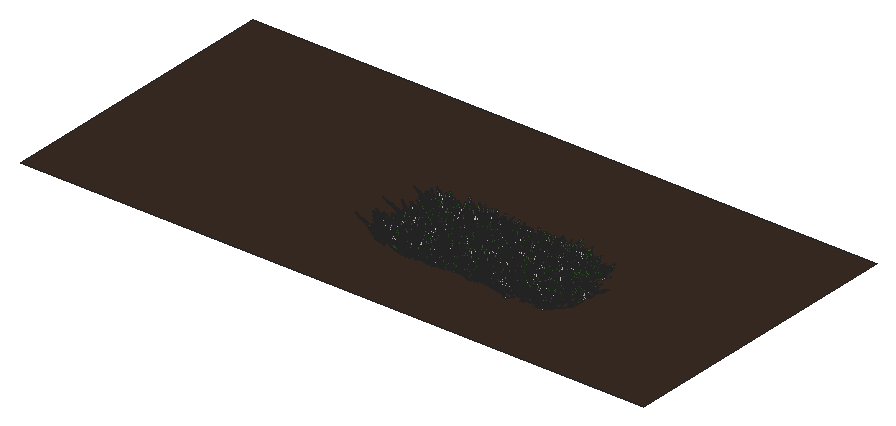
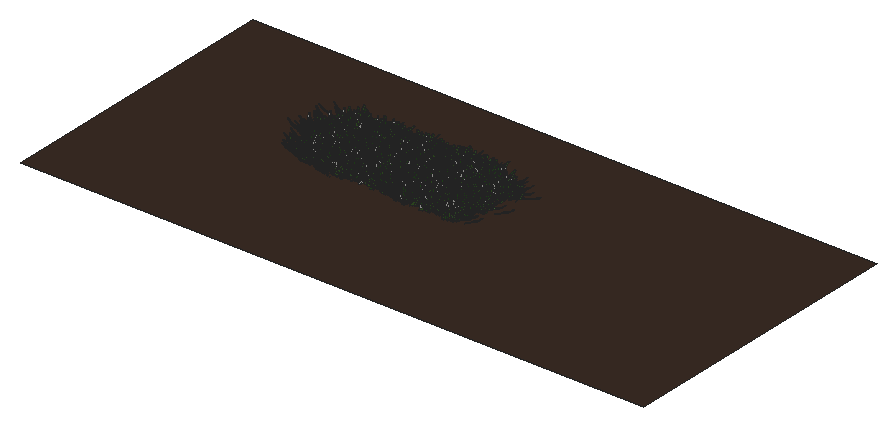
# SketchUp Ruby script. Lengths in inches.
U = 1.inch
M = Sketchup.active_model
def pt(a) = Geom::Point3d.new(a.map { |v| v * U })
def face(e, loops, mat)
  f = e.add_face(loops[0].map { |a| pt(a) })
  loops[1..].each { |l| e.add_face(l.map { |a| pt(a) }).erase! }
  f.material = f.back_material = mat if mat
  f
end
# faces: each face lists its corners as indices into pts; further lists are holes
def faces(e, pts, list, mat = nil) = list.each { |f| face(e, (f[0].is_a?(Array) ? f : [f]).map { |l| l.map { |i| pts[i] } }, mat) }
# xy, xz, yz: faces in a plane at the given z, y or x. An outline is a flat list of corners, or four numbers for a rectangle; further outlines are holes
def ring(l) = l.size == 4 ? [[l[0], l[1]], [l[2], l[1]], [l[2], l[3]], [l[0], l[3]]] : l.each_slice(2).to_a
def flat(e, list, mat, &to3) = list.each { |f| face(e, (f[0].is_a?(Array) ? f : [f]).map { |l| ring(l).map { |u, v| to3.(u, v) } }, mat) }
def xy(e, z, list, mat = nil) = flat(e, list, mat) { |x, y| [x, y, z] }
def xz(e, y, list, mat = nil) = flat(e, list, mat) { |x, z| [x, y, z] }
def yz(e, x, list, mat = nil) = flat(e, list, mat) { |y, z| [x, y, z] }
def lines(e, pts, list) = list.each { |a, b| e.add_line(pt(pts[a]), pt(pts[b])) }
# prism: a flat outline (further loops are holes) pulled along v
def prism(e, loops, v, mat = nil)
  f = face(e, loops, mat); d = Geom::Vector3d.new(v.map { |x| x * U })
  f.pushpull(f.normal.samedirection?(d) ? d.length : -d.length)
end
def box(e, o, s, mat = nil) = prism(e, [[o, [o[0] + s[0], o[1], o[2]], [o[0] + s[0], o[1] + s[1], o[2]], [o[0], o[1] + s[1], o[2]]]], [0, 0, s[2]], mat)
def at(x, y, z, deg = 0) = Geom::Transformation.translation(pt([x, y, z])) * Geom::Transformation.rotation(ORIGIN, Z_AXIS, deg.degrees)
def axes(o, x, y, z) = Geom::Transformation.new([*x, 0, *y, 0, *z, 0, *pt(o).to_a, 1])
def part(name) = M.definitions.add(name)
# library, detail: a bought-in or finely detailed component or shape, given as its bounding box
def library(name, o, s) = part(name).tap { |d| box(d.entities, o, s) }
def detail(e, o, s) = box(e.add_group.entities, o, s)
def put(e, d, t, mat = nil) = e.add_instance(d, t).tap { |i| i.material = mat if mat }
def group(e, t, mat = nil) = e.add_group.tap { |g| g.transformation = t; g.material = mat if mat }.entities
root = M.entities
M.materials.add("Material82").color = [68, 110, 58]
M.materials.add("Material83").color = [48, 90, 38]
M.materials.add("Material84").color = [68, 110, 48]
M.materials.add("Material85").color = [48, 90, 48]
M.materials.add("Material86").color = [58, 110, 58]
M.materials.add("Material87").color = [58, 90, 38]
M.materials.add("Material88").color = [68, 100, 58]
M.materials.add("Material89").color = [48, 100, 38]
M.materials.add("top-soil").color = [58, 44, 36]
c1 = part("grass00")
p = [[-0.6875,0.15,0],[-0.56,0.08,5.52],[-0.04,0.03,2.76],[0.48,-0.02,0],[0.35,-0.02,5.52],[-0.1,-0.14,5.52],
  [-0.12,0.65,8.37],[-0.42,0.65,8.37]]
faces(c1.entities,p,[[0,1,2,3],[3,2,4],[1,5,2],[5,4,2],[1,6,5],[4,5,6],[7,6,1]])
c2 = part("Group16\#1")
put(c2.entities,c1,axes([1.44,-0.61,-0.01],[0.05352,0.12609,0],[-0.10704,0.04543,0.07239],[0.06664,-0.02828,0.11628]),"Material85")
put(c2.entities,c1,axes([0.76,-0.15,-0.01],[0.04676,0.24062,0],[-0.23162,0.04501,0.06642],[0.0652,-0.01267,0.23595]),"Material82")
put(c2.entities,c1,axes([0.79,0.01,-0.01],[-0.00606,0.34651,0],[-0.34381,-0.00602,0.0432],[0.04319,0.00076,0.34386]))
put(c2.entities,c1,axes([1,0.23,-0.01],[-0.07192,0.31144,0],[-0.28722,-0.06632,0.1236],[0.12043,0.02781,0.29478]),"Material84")
put(c2.entities,c1,axes([1.66,0.77,-0.01],[-0.13828,0.29651,0],[-0.21551,-0.1005,0.22471],[0.20365,0.09498,0.23779]),"Material89")
put(c2.entities,c1,axes([0.6875,0.52,-0.01],[-0.18126,0.24051,0],[-0.22746,-0.17142,0.09788],[0.07817,0.05891,0.28481]),"Material84")
put(c2.entities,c1,axes([0.68,0.78,-0.01],[-0.215,0.18688,0],[-0.12385,-0.14248,0.21334],[0.13995,0.16101,0.18878]),"Material82")
put(c2.entities,c1,axes([0.56,1,-0.01],[-0.13756,0.07624,0],[-0.06159,-0.11112,0.0927],[0.04494,0.08108,0.12705]),"Material84")
put(c2.entities,c1,axes([0.2,0.64,-0.01],[-0.23729,0.07254,0],[-0.05711,-0.18681,0.153],[0.04473,0.14632,0.19535]),"Material89")
put(c2.entities,c1,axes([0.0625,0.72,-0.01],[-0.28874,0.02525,0],[-0.02179,-0.24916,0.14647],[0.01276,0.14591,0.25012]),"Material82")
put(c2.entities,c1,axes([-0.08,0.62,-0.01],[-0.34089,-0.04187,0],[0.03255,-0.26504,0.216],[-0.02633,0.21439,0.26703]),"Material89")
put(c2.entities,c1,axes([-0.34,0.98,-0.01],[-0.14314,-0.0493,0],[0.04397,-0.12769,0.06843],[-0.02228,0.0647,0.13505]),"Material89")
put(c2.entities,c1,axes([-0.87,1.45,-0.01],[-0.23488,-0.14114,0],[0.13761,-0.22901,0.06087],[-0.03135,0.05217,0.26717]))
put(c2.entities,c1,axes([-0.72,0.77,-0.01],[-0.14208,-0.13251,0],[0.07209,-0.0773,0.16301],[-0.11118,0.11922,0.1057]),"Material89")
put(c2.entities,c1,axes([-0.62,0.43,-0.01],[-0.14845,-0.21203,0],[0.18654,-0.13061,0.12304],[-0.10079,0.07057,0.22772]),"Material82")
put(c2.entities,c1,axes([-0.68,0.29,-0.01],[-0.13639,-0.32136,0],[0.31723,-0.13464,0.05579],[-0.05136,0.0218,0.34462]),"Material83")
put(c2.entities,c1,axes([-0.64,0.125,-0.01],[-0.0458,-0.23569,0],[0.22124,-0.043,0.08276],[-0.08124,0.01579,0.22538]),"Material86")
put(c2.entities,c1,axes([-1.6,-0.03,-0.01],[0.00576,-0.32897,0],[0.27526,0.00482,0.18018],[-0.18015,-0.00315,0.2753]),"Material84")
put(c2.entities,c1,axes([-1.36,-0.31,-0.01],[0.05718,-0.24765,0],[0.18172,0.04196,0.17267],[-0.16825,-0.03885,0.1865]),"Material89")
put(c2.entities,c1,axes([-1.54,-0.72,-0.01],[0.06537,-0.14017,0],[0.13555,0.06321,0.03939],[-0.0357,-0.01665,0.14956]))
put(c2.entities,c1,axes([-1.19,-0.9,-0.01],[0.09597,-0.12735,0],[0.11214,0.08451,0.07557],[-0.06035,-0.04548,0.14042]),"Material88")
put(c2.entities,c1,axes([-0.47,-0.54,-0.01],[0.11588,-0.10072,0],[0.0618,0.0711,0.12124],[-0.07953,-0.0915,0.0942]))
put(c2.entities,c1,axes([-0.47,-0.84,-0.01],[0.11927,-0.0661,0],[0.06603,0.11913,0.00646],[-0.00313,-0.00565,0.13621]),"Material84")
put(c2.entities,c1,axes([-0.38,-1.24,-0.01],[0.28037,-0.08571,0],[0.0618,0.20215,0.20315],[-0.05939,-0.19428,0.21139]),"Material88")
put(c2.entities,c1,axes([-0.06,-0.66,-0.01],[0.22719,-0.01987,0],[0.01247,0.14255,0.17758],[-0.01547,-0.17691,0.1431]),"Material87")
put(c2.entities,c1,axes([0.11,-0.89,-0.01],[0.14882,0.01828,0],[-0.01058,0.08611,0.12229],[0.01491,-0.12138,0.08676]),"Material85")
put(c2.entities,c1,axes([0.25,-0.72,-0.01],[0.20481,0.07053,0],[-0.06206,0.18022,0.10291],[0.03351,-0.0973,0.1906]),"Material85")
put(c2.entities,c1,axes([0.85,-1.42,-0.01],[0.16481,0.09904,0],[-0.09472,0.15762,0.05616],[0.02893,-0.04814,0.18389]),"Material84")
put(c2.entities,c1,axes([1.01,-1.09,-0.01],[0.21858,0.20385,0],[-0.17495,0.1876,0.15339],[0.10462,-0.11218,0.25652]),"Material89")
put(c2.entities,c1,axes([1.01,-0.71,-0.01],[0.08733,0.12473,0],[-0.06445,0.04512,0.13037],[0.1068,-0.07477,0.07867]),"Material85")
c3 = part("Group15\#1")
put(c3.entities,c2,at(0,0,0))
c4 = part("3darcstudiotree_grass00\#1")
put(c4.entities,c3,at(0,0,0))
xy(root,-34.17,[[1644.93,281.03,1887.96,394.45]],"top-soil")
put(root,c4,axes([1812.29,310.03,-34.17],[-3.54698,0.73807,0],[-1.81276,-1.35492,-0.01893],[-0.04162,-0.0311,1.37131]))
put(root,c4,axes([1777.81,310.98,-34.17],[-3.86461,-0.59074,0],[1.45311,-1.4785,-0.05586],[0.12869,-0.13094,1.92103]))
put(root,c4,axes([1823.08,311.05,-34.17],[-0.38971,1.40175,0],[-3.70548,-0.16023,-0.02456],[-0.14917,-0.00645,1.70727]))
put(root,c4,axes([1787.3,311.33,-34.17],[-3.70591,-0.99796,0],[1.87776,-1.08451,-0.01838],[0.07513,-0.04339,1.80866]))
put(root,c4,axes([1811.92,311.37,-34.17],[2.84839,1.04367,0],[-2.27167,0.96426,-0.03885],[-0.20657,0.08768,1.95422]))
put(root,c4,axes([1798,311.6875,-34.17],[-1.7758,-1.16797,0],[3.11451,-0.73649,-0.04451],[0.21848,-0.05166,1.55797]))
put(root,c4,axes([1773.88,311.53,-34.17],[2.01516,1.65729,0],[-3.55056,0.67146,-0.00104],[-0.005,0.00095,1.58037]))
put(root,c4,axes([1767.14,312.05,-34.17],[-0.55616,-1.38612,0],[4.6364,-0.28933,-0.05346],[0.22148,-0.01382,1.47567]))
put(root,c4,axes([1816.37,312.35,-34.17],[3.94842,-0.68884,0],[1.45256,1.29494,-0.00969],[0.01982,0.01767,1.36001]))
put(root,c4,axes([1803.41,312.01,-34.17],[-3.65792,-0.8597,0],[1.995,-1.32021,-0.01663],[0.05672,-0.03754,1.94585]))
put(root,c4,axes([1784.11,312.25,-34.17],[-2.06404,-1.37727,0],[3.69374,-0.86095,-0.04139],[0.20463,-0.0477,1.84708]))
put(root,c4,axes([1794.42,312.16,-34.17],[-3.29266,-0.34854,0],[0.95777,-1.40726,-0.03217],[0.05606,-0.08237,1.86146]))
put(root,c4,axes([1782.4375,312.97,-34.17],[3.44047,-0.2055,0],[0.68194,1.77564,-0.05863],[0.04271,0.1112,1.66018]))
put(root,c4,axes([1823.62,313.17,-34.17],[3.33641,-0.4539,0],[1.10224,1.26009,-0.03311],[0.06709,0.0767,1.57439]))
put(root,c4,axes([1809.42,313.4,-34.17],[4.05026,0.33604,0],[-0.7921,1.48485,-0.04482],[-0.0484,0.09073,1.51278]))
put(root,c4,axes([1788.85,312.91,-34.17],[-1.23007,1.60855,0],[-3.72331,-0.44283,-0.01363],[-0.06328,-0.00753,1.41312]))
put(root,c4,axes([1805.98,313.31,-34.17],[-4.03093,-0.26709,0],[0.61626,-1.44652,-0.01654],[0.01865,-0.04378,1.89711]))
put(root,c4,axes([1793.05,313.83,-34.17],[1.95292,1.06951,0],[-2.86765,0.8144,-0.02117],[-0.10996,0.03123,1.69559]))
put(root,c4,axes([1815.95,314.28,-34.17],[4.38423,0.4309,0],[-1.14012,1.80418,-0.03274],[-0.03634,0.0575,1.62193]))
put(root,c4,axes([1797.91,314.1,-34.17],[-2.45174,-1.03973,0],[2.50397,-0.91832,-0.03633],[0.18002,-0.06602,1.73438]))
put(root,c4,axes([1777.67,314.16,-34.17],[-1.89614,-1.52378,0],[3.69892,-0.71587,-0.01008],[0.04587,-0.00888,1.566]))
put(root,c4,axes([1773.97,314.51,-34.17],[3.35774,0.54146,0],[-1.57719,1.52117,-0.03911],[-0.07127,0.06874,1.50402]))
put(root,c4,axes([1766.31,314.1,-34.17],[-3.39635,0.60304,0],[-1.8174,-1.59194,-0.05685],[-0.1325,-0.11606,1.88376]))
put(root,c4,axes([1781.73,315.21,-34.17],[3.39282,-0.2362,0],[0.75884,1.6953,-0.03701],[0.03902,0.08718,1.98432]))
put(root,c4,axes([1804.04,315.28,-34.17],[0.6087,1.43701,0],[-3.38203,0.22281,-0.00028],[-0.00164,0.00011,1.50491]))
put(root,c4,axes([1809.99,316.08,-34.17],[3.17929,-0.7211,0],[2.23361,1.53163,-0.03788],[0.07878,0.05402,1.40078]))
put(root,c4,axes([1798.57,315.53,-34.17],[2.01819,1.66422,0],[-3.45385,0.65143,-0.02212],[-0.1358,0.02561,1.95299]))
put(root,c4,axes([1792.77,315.7,-34.17],[-0.16089,1.57179,0],[-4.27524,-0.06806,-0.04298],[-0.25282,-0.00402,1.88799]))
put(root,c4,axes([1814.92,315.95,-34.17],[-3.05635,-0.6343,0],[1.70161,-1.2752,-0.01604],[0.05188,-0.03888,1.9024]))
put(root,c4,axes([1771.19,316.11,-34.17],[0.91536,1.26151,0],[-4.37209,0.4934,-0.02742],[-0.14974,0.0169,1.93645]))
put(root,c4,axes([1787.6,316.09,-34.17],[-3.8828,0.51827,0],[-1.09306,-1.27365,-0.02484],[-0.06133,-0.07146,1.96802]))
put(root,c4,axes([1777.19,316.45,-34.17],[2.24895,1.38406,0],[-3.92977,0.99312,-0.02786],[-0.13256,0.0335,1.9768]))
put(root,c4,axes([1822.07,316.62,-34.17],[-3.21256,-1.12789,0],[2.70503,-1.19832,-0.03256],[0.11538,-0.05111,1.62483]))
put(root,c4,axes([1765.55,316.28,-34.17],[-2.03127,1.47153,0],[-3.87167,-0.83121,-0.05406],[-0.22119,-0.04749,1.53936]))
put(root,c4,axes([1761.34,316.375,-34.17],[-3.53362,0.69285,0],[-1.78137,-1.413,-0.01143],[-0.02296,-0.01821,1.35283]))
put(root,c4,axes([1817.82,317.78,-34.17],[4.62104,-0.01455,0],[0.03483,1.71996,-0.00522],[0.00018,0.00901,1.42947]))
put(root,c4,axes([1776.38,317.75,-34.17],[-3.41262,-0.98405,0],[2.00346,-1.0806,-0.03203],[0.14502,-0.07822,1.95145]))
put(root,c4,axes([1810.85,318.16,-34.17],[4.2068,0.84458,0],[-2.08885,1.6182,-0.01612],[-0.03432,0.02659,1.61949]))
put(root,c4,axes([1772.96,317.9375,-34.17],[-3.8851,-1.03716,0],[2.44189,-1.42264,-0.04034],[0.11257,-0.06558,1.62559]))
put(root,c4,axes([1793.55,318.31,-34.17],[4.5376,0.13529,0],[-0.33368,1.74059,-0.04634],[-0.02094,0.10925,1.98901]))
put(root,c4,axes([1762.86,318.48,-34.17],[3.81611,-0.29546,0],[0.81359,1.63432,-0.02697],[0.02626,0.05275,1.59996]))
put(root,c4,axes([1788.64,318.49,-34.17],[4.2001,-0.13479,0],[0.33266,1.61217,-0.01977],[0.00834,0.04041,1.59866]))
put(root,c4,axes([1798.32,318.43,-34.17],[4.12561,0.29265,0],[-0.72369,1.58676,-0.03729],[-0.0346,0.07587,1.60628]))
put(root,c4,axes([1823.875,317.94,-34.17],[-4.01452,0.69277,0],[-1.67449,-1.50916,-0.02625],[-0.04914,-0.04429,1.46233]))
put(root,c4,axes([1806.1875,318.46,-34.17],[-3.3453,-1.30601,0],[3.28392,-1.30825,-0.03717],[0.14464,-0.05762,1.93537]))
put(root,c4,axes([1767.78,318.38,-34.17],[-0.84571,1.33613,0],[-3.59715,-0.35412,-0.00012],[-0.00056,-0.00006,1.39497]))
put(root,c4,axes([1784.96,318.8125,-34.17],[1.55645,1.18195,0],[-3.2541,0.66647,-0.04821],[-0.21297,0.04362,1.36797]))
put(root,c4,axes([1815.88,319.5,-34.17],[0.41929,-1.46273,0],[4.6699,0.2082,-0.01256],[0.06761,0.00301,1.90836]))
put(root,c4,axes([1761.02,319.51,-34.17],[1.28441,1.48375,0],[-3.48852,0.46968,-0.04031],[-0.24472,0.03295,1.77227]))
put(root,c4,axes([1806.37,319.89,-34.17],[-1.63649,-1.29377,0],[3.38922,-0.66676,-0.00448],[0.02699,-0.00531,1.90991]))
put(root,c4,axes([1800.66,319.75,-34.17],[-2.13819,1.22316,0],[-3.167,-0.86103,-0.02321],[-0.1127,-0.03064,1.70026]))
put(root,c4,axes([1775.84,320.25,-34.17],[-2.39621,-0.97294,0],[2.61152,-1.00033,-0.02073],[0.08443,-0.03234,1.5494]))
put(root,c4,axes([1810.52,320.59,-34.17],[3.58142,-0.447,0],[1.06233,1.32378,-0.04021],[0.07095,0.08841,1.5432]))
put(root,c4,axes([1783.1,320.74,-34.17],[4.64305,-0.03413,0],[0.08366,1.7702,-0.03615],[0.00311,0.0658,1.55355]))
put(root,c4,axes([1789.91,320.08,-34.17],[-4.51566,0.3438,0],[-0.75132,-1.53478,-0.00152],[-0.00137,-0.0028,1.41339]))
put(root,c4,axes([1771.98,320.93,-34.17],[2.30193,-1.12166,0],[3.41965,1.0915,-0.0352],[0.15447,0.0493,1.86157]))
put(root,c4,axes([1792.92,320.59,-34.17],[-3.57945,0.04189,0],[-0.11544,-1.5341,-0.02538],[-0.0045,-0.05977,1.74242]))
put(root,c4,axes([1768.37,321.05,-34.17],[3.76479,0.94059,0],[-2.16386,1.34705,-0.03414],[-0.08584,0.05343,1.42377]))
put(root,c4,axes([1822.15,320.78,-34.17],[-3.59955,0.15303,0],[-0.4164,-1.52331,-0.01956],[-0.01422,-0.05201,1.97453]))
put(root,c4,axes([1777.96,321.72,-34.17],[1.47145,-1.32607,0],[3.01918,0.52105,-0.00213],[0.01031,0.00178,1.30651]))
put(root,c4,axes([1782.31,321.95,-34.17],[2.13019,1.09948,0],[-3.08878,0.93074,-0.0123],[-0.05365,0.01617,1.59876]))
put(root,c4,axes([1826.06,322.0625,-34.17],[-2.71685,-1.17622,0],[2.71806,-0.97644,-0.02128],[0.11147,-0.04005,1.95268]))
put(root,c4,axes([1766.53,321.84,-34.17],[-1.39977,1.36626,0],[-3.55438,-0.56636,-0.02451],[-0.1313,-0.02092,1.66036]))
put(root,c4,axes([1810.35,322.68,-34.17],[3.81863,-0.53813,0],[1.40932,1.55539,-0.0155],[0.0332,0.03664,1.9985]))
put(root,c4,axes([1789.17,321.92,-34.17],[-3.79382,0.9598,0],[-2.14839,-1.32076,-0.01729],[-0.051,-0.03135,1.62898]))
put(root,c4,axes([1820.74,322.59,-34.17],[-3.51388,-0.90483,0],[2.14031,-1.29273,-0.0556],[0.17294,-0.10445,1.66946]))
put(root,c4,axes([1770.35,323.23,-34.17],[2.94171,-1.11183,0],[3.18535,1.31078,-0.03986],[0.13301,0.05473,1.66404]))
put(root,c4,axes([1795.24,322.85,-34.17],[2.7006,1.1614,0],[-2.43909,0.8821,-0.03804],[-0.19893,0.07194,1.7602]))
put(root,c4,axes([1799.84,322.94,-34.17],[-3.12186,-1.16816,0],[2.84193,-1.18123,-0.00166],[0.00643,-0.00267,1.74215]))
put(root,c4,axes([1815.9375,322.79,-34.17],[-2.88569,0.96312,0],[-2.81786,-1.31311,-0.05904],[-0.17262,-0.08044,1.47981]))
put(root,c4,axes([1805.17,322.8,-34.17],[-3.14808,1.22755,0],[-2.57668,-1.02773,-0.03762],[-0.14164,-0.05649,1.47105]))
put(root,c4,axes([1781.68,323.95,-34.17],[1.01985,1.24994,0],[-3.27441,0.41552,-0.0339],[-0.22651,0.02874,1.80984]))
put(root,c4,axes([1771.75,324.76,-34.17],[-0.23596,-1.70659,0],[3.32039,-0.0714,-0.01049],[0.06174,-0.00133,1.4693]))
put(root,c4,axes([1815.07,324.7,-34.17],[-0.79946,-1.53657,0],[4.27905,-0.34626,-0.03341],[0.18605,-0.01506,1.86102]))
put(root,c4,axes([1766.97,324.79,-34.17],[3.51248,0.23364,0],[-0.65189,1.52422,-0.03005],[-0.02625,0.06139,1.54341]))
put(root,c4,axes([1810.48,324.54,-34.17],[-3.28059,-1.08182,0],[2.91353,-1.37413,-0.04137],[0.10673,-0.05034,1.36909]))
put(root,c4,axes([1789.05,324.66,-34.17],[2.36553,1.18037,0],[-3.06807,0.95629,-0.02315],[-0.10187,0.03175,1.64391]))
put(root,c4,axes([1799.01,324.88,-34.17],[2.46344,0.86677,0],[-2.31784,1.02455,-0.00625],[-0.02756,0.01218,1.72796]))
put(root,c4,axes([1795.2,324.75,-34.17],[2.29641,1.07421,0],[-2.57105,0.85483,-0.04117],[-0.19383,0.06444,1.55213]))
put(root,c4,axes([1778.1,324.66,-34.17],[-2.89048,1.44179,0],[-2.90546,-0.90593,-0.0043],[-0.02277,-0.0071,1.8735]))
put(root,c4,axes([1805,324.94,-34.17],[0.67214,1.30105,0],[-3.68417,0.29602,-0.04728],[-0.27019,0.02171,1.64346]))
put(root,c4,axes([1825.78,325.4,-34.17],[-4.08837,-0.48406,0],[1.24556,-1.63618,-0.01736],[0.02056,-0.027,1.33702]))
put(root,c4,axes([1823.08,325.37,-34.17],[-2.8527,1.28628,0],[-3.36111,-1.15935,-0.03347],[-0.14409,-0.0497,1.91416]))
put(root,c4,axes([1776.62,326.04,-34.17],[4.59378,0.22046,0],[-0.54654,1.77125,-0.0359],[-0.02405,0.07793,1.88046]))
put(root,c4,axes([1818.01,326.41,-34.17],[1.74244,1.18271,0],[-3.27168,0.74965,-0.03711],[-0.19162,0.04391,1.69359]))
put(root,c4,axes([1823.29,326.76,-34.17],[-1.03972,-1.40109,0],[4.3795,-0.50546,-0.04795],[0.2061,-0.02379,1.53186]))
put(root,c4,axes([1782.64,326.58,-34.17],[-2.79426,-0.70511,0],[1.77672,-1.09506,-0.02395],[0.07288,-0.04492,1.39534]))
put(root,c4,axes([1772.66,326.76,-34.17],[-2.68837,-0.8629,0],[2.90522,-1.40773,-0.04334],[0.1065,-0.05161,1.34295]))
put(root,c4,axes([1801.26,327.31,-34.17],[2.12809,-1.0558,0],[3.61722,1.13396,-0.06111],[0.24603,0.07713,1.78135]))
put(root,c4,axes([1787.32,327.42,-34.17],[0.0983,-1.39772,0],[3.56781,0.03903,-0.00183],[0.01012,0.00011,1.48199]))
put(root,c4,axes([1765.74,327.59,-34.17],[4.07348,0.57799,0],[-1.18057,1.29405,-0.01256],[-0.02962,0.03247,1.82155]))
put(root,c4,axes([1808.97,327.39,-34.17],[-4.0386,-0.4374,0],[0.94795,-1.36128,-0.02848],[0.0516,-0.0741,1.83531]))
put(root,c4,axes([1793.69,327.45,-34.17],[1.35175,1.46561,0],[-4.38115,0.62846,-0.0524],[-0.19286,0.02766,1.36852]))
put(root,c4,axes([1804.03,327.56,-34.17],[0.48824,1.58889,0],[-4.56618,0.21822,-0.01569],[-0.06712,0.00321,1.48562]))
put(root,c4,axes([1807.26,328.5,-34.17],[3.86781,0.52244,0],[-1.13731,1.30954,-0.02009],[-0.0432,0.04974,1.7458]))
put(root,c4,axes([1773.41,328.63,-34.17],[4.03922,-0.03156,0],[0.07296,1.45219,-0.01855],[0.00258,0.0513,1.93628]))
put(root,c4,axes([1817.21,328.19,-34.17],[-1.29956,1.24249,0],[-3.63161,-0.59077,-0.01866],[-0.09119,-0.01483,1.55626]))
put(root,c4,axes([1784.39,328.29,-34.17],[-4.29389,-0.13256,0],[0.34176,-1.72178,-0.05117],[0.01874,-0.09441,1.54048]))
put(root,c4,axes([1811.1875,328.66,-34.17],[-2.84597,-0.98358,0],[2.28129,-1.02662,-0.01406],[0.06335,-0.02851,1.77353]))
put(root,c4,axes([1766.58,329.28,-34.17],[2.50193,-0.87133,0],[2.32937,1.04026,-0.01409],[0.05813,0.02596,1.64399]))
put(root,c4,axes([1790.08,328.99,-34.17],[-4.49069,-0.28234,0],[0.61208,-1.5141,-0.05098],[0.04605,-0.11392,1.67187]))
put(root,c4,axes([1778.37,329.6,-34.17],[4.61322,-0.12203,0],[0.30512,1.79396,-0.00473],[0.00139,0.00815,1.49489]))
put(root,c4,axes([1793.41,329.34,-34.17],[-2.62594,-1.45094,0],[3.42478,-0.964,-0.01802],[0.06257,-0.01761,1.345]))
put(root,c4,axes([1821.64,329,-34.17],[-1.19351,1.65501,0],[-3.6228,-0.40633,-0.01558],[-0.10093,-0.01132,1.90128]))
put(root,c4,axes([1798,329.74,-34.17],[3.25093,0.54248,0],[-1.41803,1.32165,-0.02719],[-0.07494,0.06985,1.929]))
put(root,c4,axes([1762.04,329.53,-34.17],[-3.58514,0.47051,0],[-1.41535,-1.67729,-0.02244],[-0.03437,-0.04073,1.62972]))
put(root,c4,axes([1772.52,330.47,-34.17],[4.08766,0.51132,0],[-1.24704,1.55051,-0.00141],[-0.00269,0.00335,1.95289]))
put(root,c4,axes([1820.92,330.72,-34.17],[0.81424,-1.34129,0],[3.64589,0.34423,-0.00366],[0.01919,0.00181,1.51551]))
put(root,c4,axes([1812.4375,330.89,-34.17],[3.6343,-0.40762,0],[1.19135,1.65202,-0.03545],[0.05267,0.07304,1.77295]))
put(root,c4,axes([1798.01,330.42,-34.17],[-0.25702,1.50589,0],[-4.4334,-0.11768,-0.01753],[-0.09867,-0.00262,1.87889]))
put(root,c4,axes([1817.55,330.55,-34.17],[-3.92506,-0.07313,0],[0.21494,-1.79423,-0.03065],[0.00834,-0.06965,1.9691]))
put(root,c4,axes([1790.5625,331.07,-34.17],[3.46346,0.58344,0],[-1.61207,1.48838,-0.00364],[-0.00911,0.00841,1.96053]))
put(root,c4,axes([1766.46,331.8,-34.17],[1.7154,-1.15643,0],[3.09768,0.71465,-0.02347],[0.14538,0.03354,1.9305]))
put(root,c4,axes([1804.35,331.23,-34.17],[-0.11554,1.45354,0],[-4.02615,-0.04978,-0.04067],[-0.20655,-0.00255,1.53414]))
put(root,c4,axes([1785.1,331.38,-34.17],[0.845,1.27042,0],[-4.02841,0.41673,-0.05161],[-0.24313,0.02515,1.52021]))
put(root,c4,axes([1795.58,331.61,-34.17],[-4.23196,-0.66829,0],[1.43136,-1.40974,-0.04264],[0.09281,-0.09141,1.69007]))
put(root,c4,axes([1777.54,331.44,-34.17],[-4.40755,0.3662,0],[-0.80873,-1.51388,-0.00142],[-0.00162,-0.00303,1.63114]))
put(root,c4,axes([1804.58,332.75,-34.17],[2.10607,-1.53284,0],[3.55653,0.76,-0.00988],[0.05409,0.01156,1.88737]))
put(root,c4,axes([1773.85,332.89,-34.17],[1.61408,-1.6002,0],[4.35972,0.68394,-0.04298],[0.19186,0.0301,1.68954]))
put(root,c4,axes([1820.31,333.02,-34.17],[-3.98486,0.06108,0],[-0.1339,-1.35868,-0.04521],[-0.01298,-0.1317,1.91035]))
put(root,c4,axes([1808.71,333.45,-34.17],[-0.39879,-1.78911,0],[3.98788,-0.13825,-0.04765],[0.27848,-0.00965,1.76037]))
put(root,c4,axes([1788.9375,333.45,-34.17],[2.70315,0.92974,0],[-3.09727,1.40055,-0.01764],[-0.05733,0.02592,1.74631]))
put(root,c4,axes([1801.375,334.01,-34.17],[3.47556,-0.63984,0],[1.81232,1.53108,-0.02938],[0.06383,0.05392,1.64954]))
put(root,c4,axes([1794.6,334.04,-34.17],[2.88826,-0.72218,0],[1.92215,1.1956,-0.03299],[0.1167,0.07259,1.77748]))
put(root,c4,axes([1816.18,333.52,-34.17],[-4.37429,0.70017,0],[-1.56113,-1.51689,-0.01879],[-0.03338,-0.03243,1.46955]))
put(root,c4,axes([1777.66,333.57,-34.17],[-3.74567,1.07998,0],[-2.52019,-1.35944,-0.03994],[-0.14532,-0.07839,1.97331]))
put(root,c4,axes([1768.1,333.84,-34.17],[-1.51727,1.49458,0],[-3.30202,-0.52136,-0.01826],[-0.09361,-0.01478,1.47196]))
put(root,c4,axes([1783.24,333.9,-34.17],[-2.53173,1.21264,0],[-2.8931,-0.93942,-0.04557],[-0.23211,-0.07537,1.85346]))
put(root,c4,axes([1817.11,335.24,-34.17],[3.99314,-0.58395,0],[1.40862,1.49812,-0.01564],[0.03379,0.03593,1.88746]))
put(root,c4,axes([1776.2,335.24,-34.17],[2.23301,-1.20393,0],[2.80312,0.80861,-0.02877],[0.133,0.03837,1.49076]))
put(root,c4,axes([1806.23,335.05,-34.17],[3.03872,1.12896,0],[-3.11924,1.30579,-0.01047],[-0.04051,0.01696,1.92288]))
put(root,c4,axes([1822.67,335.05,-34.17],[-2.41013,-1.27132,0],[2.91819,-0.86042,-0.02089],[0.0972,-0.02866,1.58683]))
put(root,c4,axes([1764.97,334.86,-34.17],[-1.21919,1.74404,0],[-3.47137,-0.37742,-0.03305],[-0.15949,-0.01734,1.35106]))
put(root,c4,axes([1787.14,335.3125,-34.17],[4.18586,0.29447,0],[-0.62505,1.38186,-0.04495],[-0.05854,0.12943,1.97854]))
put(root,c4,axes([1794.46,335.49,-34.17],[1.93247,1.08024,0],[-2.71059,0.75417,-0.03223],[-0.14585,0.04058,1.37708]))
put(root,c4,axes([1781.44,335.86,-34.17],[-2.49297,-0.95003,0],[2.84759,-1.16217,-0.03177],[0.13042,-0.05323,1.8145]))
put(root,c4,axes([1772.33,336.1,-34.17],[3.82297,0.44431,0],[-0.93883,1.25636,-0.026],[-0.04711,0.06304,1.59572]))
put(root,c4,axes([1808.93,335.94,-34.17],[-3.75498,0.92244,0],[-1.75834,-1.11323,-0.01072],[-0.04199,-0.02659,1.84718]))
put(root,c4,axes([1798.49,336.12,-34.17],[0.4621,1.41992,0],[-4.03416,0.20419,-0.0516],[-0.33532,0.01697,1.99718]))
put(root,c4,axes([1784.75,337.27,-34.17],[-3.18702,-0.48311,0],[1.45771,-1.49562,-0.04802],[0.08757,-0.08985,1.54794]))
put(root,c4,axes([1778.22,337.9,-34.17],[4.11101,0.00408,0],[-0.01055,1.6533,-0.01268],[-0.00019,0.02913,1.83013]))
put(root,c4,axes([1798.45,337.57,-34.17],[-2.73846,-0.74739,0],[2.06192,-1.17502,-0.03348],[0.13147,-0.07492,1.87437]))
put(root,c4,axes([1812.44,337.86,-34.17],[-2.02199,-1.57321,0],[3.0284,-0.60536,-0.03791],[0.25064,-0.0501,1.88609]))
put(root,c4,axes([1821.6,337.55,-34.17],[-3.15684,0.83052,0],[-1.94414,-1.14932,-0.03251],[-0.12313,-0.07279,1.79208]))
put(root,c4,axes([1806.18,338.17,-34.17],[2.88281,0.64392,0],[-1.76321,1.22772,-0.02459],[-0.08623,0.06004,1.90817]))
put(root,c4,axes([1765.69,337.82,-34.17],[-0.3994,1.69229,0],[-4.36532,-0.16024,-0.02425],[-0.12976,-0.00476,1.76617]))
put(root,c4,axes([1788.57,338.35,-34.17],[-0.50603,-1.39331,0],[4.58553,-0.25902,-0.00214],[0.00976,-0.00055,1.59988]))
put(root,c4,axes([1773.0625,338.22,-34.17],[0.99401,1.39114,0],[-3.81883,0.42439,-0.02067],[-0.11338,0.0126,1.69495]))
put(root,c4,axes([1795.87,338.21,-34.17],[0.45996,1.33665,0],[-3.57607,0.19139,-0.02967],[-0.17102,0.00915,1.57371]))
put(root,c4,axes([1817.75,338.14,-34.17],[-1.48177,1.26839,0],[-3.97677,-0.72256,-0.00587],[-0.02393,-0.00435,1.47291]))
put(root,c4,axes([1781.63,339.12,-34.17],[2.466,-1.02389,0],[3.09141,1.158,-0.03691],[0.15975,0.05984,1.90749]))
put(root,c4,axes([1779.21,339.33,-34.17],[3.21693,-1.31198,0],[2.89205,1.10289,-0.03201],[0.144,0.05492,1.88682]))
put(root,c4,axes([1806.27,339.26,-34.17],[3.38308,1.28097,0],[-3.13031,1.28579,-0.04664],[-0.1697,0.06971,1.77978]))
put(root,c4,axes([1765.21,339.17,-34.17],[-3.15287,0.69435,0],[-1.94177,-1.37131,-0.05669],[-0.17259,-0.12189,1.86391]))
put(root,c4,axes([1810.15,339.26,-34.17],[-1.68767,1.14523,0],[-4.10192,-0.94014,-0.02835],[-0.11929,-0.02734,1.73088]))
